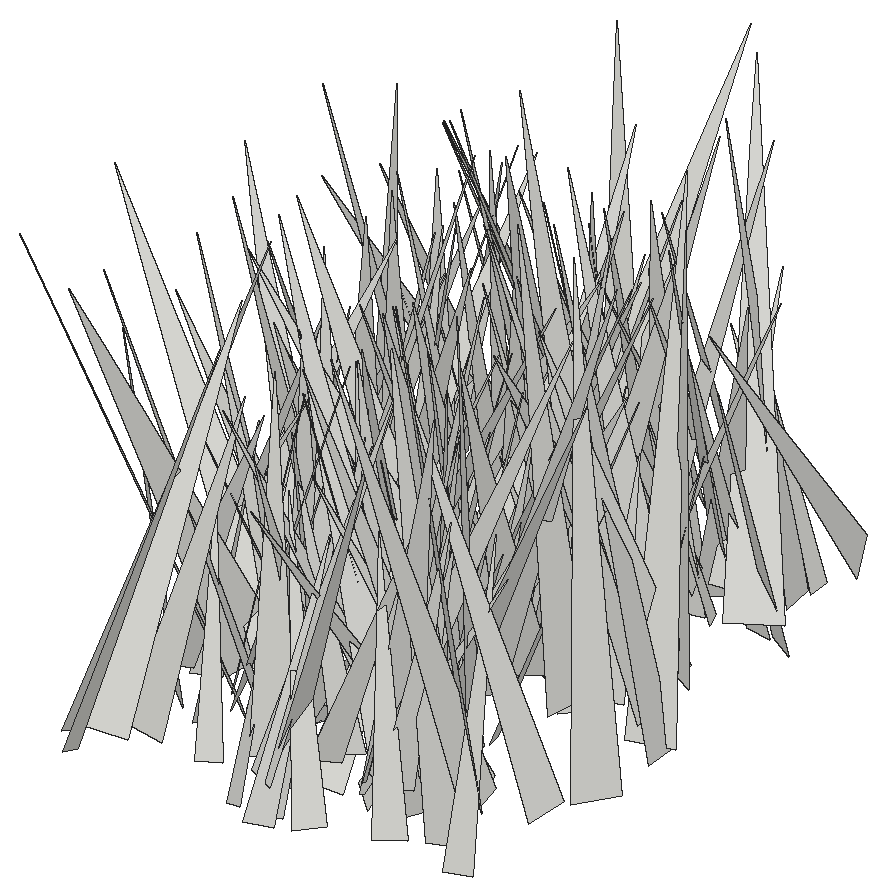
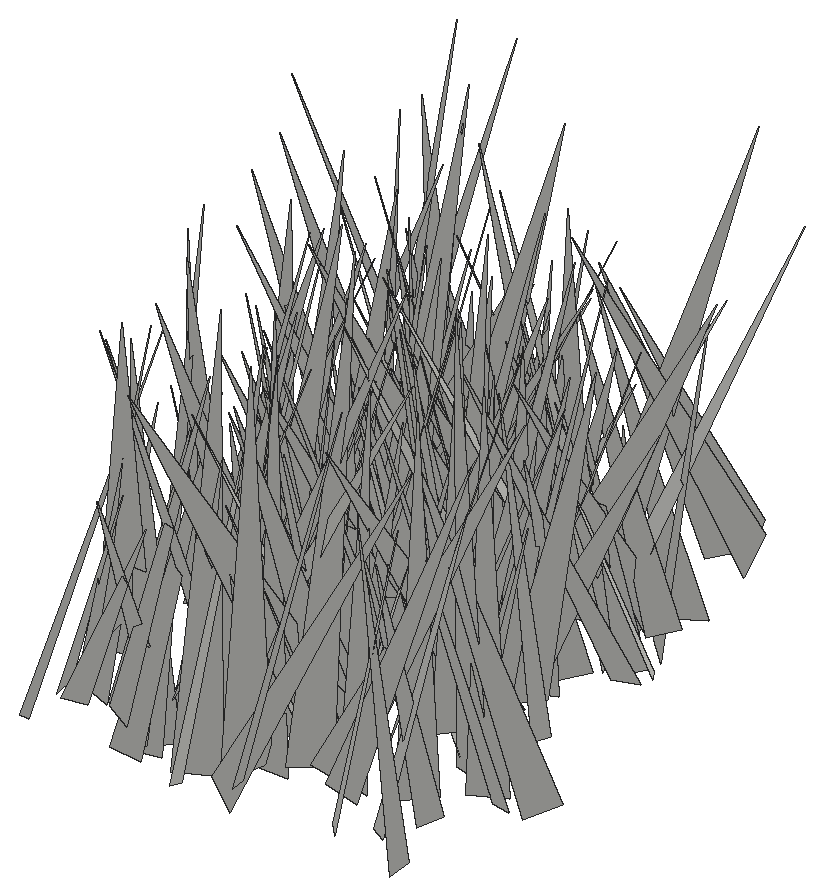
# SketchUp Ruby script. Lengths in inches.
U = 1.inch
M = Sketchup.active_model
def pt(a) = Geom::Point3d.new(a.map { |v| v * U })
def face(e, loops, mat)
  f = e.add_face(loops[0].map { |a| pt(a) })
  loops[1..].each { |l| e.add_face(l.map { |a| pt(a) }).erase! }
  f.material = f.back_material = mat if mat
  f
end
# faces: each face lists its corners as indices into pts; further lists are holes
def faces(e, pts, list, mat = nil) = list.each { |f| face(e, (f[0].is_a?(Array) ? f : [f]).map { |l| l.map { |i| pts[i] } }, mat) }
# xy, xz, yz: faces in a plane at the given z, y or x. An outline is a flat list of corners, or four numbers for a rectangle; further outlines are holes
def ring(l) = l.size == 4 ? [[l[0], l[1]], [l[2], l[1]], [l[2], l[3]], [l[0], l[3]]] : l.each_slice(2).to_a
def flat(e, list, mat, &to3) = list.each { |f| face(e, (f[0].is_a?(Array) ? f : [f]).map { |l| ring(l).map { |u, v| to3.(u, v) } }, mat) }
def xy(e, z, list, mat = nil) = flat(e, list, mat) { |x, y| [x, y, z] }
def xz(e, y, list, mat = nil) = flat(e, list, mat) { |x, z| [x, y, z] }
def yz(e, x, list, mat = nil) = flat(e, list, mat) { |y, z| [x, y, z] }
def lines(e, pts, list) = list.each { |a, b| e.add_line(pt(pts[a]), pt(pts[b])) }
# prism: a flat outline (further loops are holes) pulled along v
def prism(e, loops, v, mat = nil)
  f = face(e, loops, mat); d = Geom::Vector3d.new(v.map { |x| x * U })
  f.pushpull(f.normal.samedirection?(d) ? d.length : -d.length)
end
def box(e, o, s, mat = nil) = prism(e, [[o, [o[0] + s[0], o[1], o[2]], [o[0] + s[0], o[1] + s[1], o[2]], [o[0], o[1] + s[1], o[2]]]], [0, 0, s[2]], mat)
def at(x, y, z, deg = 0) = Geom::Transformation.translation(pt([x, y, z])) * Geom::Transformation.rotation(ORIGIN, Z_AXIS, deg.degrees)
def axes(o, x, y, z) = Geom::Transformation.new([*x, 0, *y, 0, *z, 0, *pt(o).to_a, 1])
def part(name) = M.definitions.add(name)
# library, detail: a bought-in or finely detailed component or shape, given as its bounding box
def library(name, o, s) = part(name).tap { |d| box(d.entities, o, s) }
def detail(e, o, s) = box(e.add_group.entities, o, s)
def put(e, d, t, mat = nil) = e.add_instance(d, t).tap { |i| i.material = mat if mat }
def group(e, t, mat = nil) = e.add_group.tap { |g| g.transformation = t; g.material = mat if mat }.entities
root = M.entities
c1 = part("fur_instance\#9")
p = [[0.8125,0,1.79],[0.67,-0.02,1.48],[0,-0.11,0],[0,0.11,0]]
faces(c1.entities,p,[[0,1,2,3]])
put(root,c1,axes([75.7,109.57,-28.22],[5.32416,0.8497,1.29821],[1.01973,-5.41351,-0.63884],[-1.1694,-0.85204,5.35356]))
put(root,c1,axes([79.16,99.36,-28.22],[-6.20404,3.776,0.73856],[3.82283,6.20814,0.37243],[0.43544,-0.70326,7.25325]))
put(root,c1,axes([79.8125,94.96,-28.22],[-5.60021,-5.8066,0.30959],[-5.79691,5.54128,-0.92996],[-0.45638,0.8674,8.01337]))
put(root,c1,axes([77.96,94.43,-28.22],[-3.7574,-4.18768,1.74578],[-4.4509,3.84178,-0.36412],[0.87968,1.55129,5.61445]))
put(root,c1,axes([79.72,98.95,-28.22],[-2.55985,4.83206,1.74885],[4.89019,1.69025,2.4878],[-1.579,-2.59892,4.86955]))
put(root,c1,axes([77.5,110.44,-27.1],[3.26712,2.26093,2.86418],[3.20778,-3.61207,-0.80776],[-1.73938,-2.41465,3.89016]))
put(root,c1,axes([74.52,104.19,-28.22],[4.53332,-3.78068,0.06575],[-3.6354,-4.32956,1.69931],[1.04008,1.34544,5.65304]))
put(root,c1,axes([77.53,108.27,-28.22],[-3.10311,-4.08719,0.56583],[-3.96021,3.14894,1.02739],[1.15846,-0.18348,5.02781]))
put(root,c1,axes([80.89,95.66,-27.1],[-4.85114,5.94494,0.47809],[5.69058,4.42924,2.66526],[-1.78556,-2.03568,7.19529]))
put(root,c1,axes([76.41,104.47,-28.22],[2.07468,-5.92746,1.15005],[-6.03286,-1.98482,0.6533],[0.24901,1.299,6.24598]))
put(root,c1,axes([78.66,108.61,-27.1],[-0.3519,-5.66898,0.64957],[-5.59847,0.21723,-1.13712],[-1.1029,0.70611,5.5649]))
put(root,c1,axes([76.78,106.73,-28.22],[3.97041,-1.42005,1.05601],[-1.57618,-4.01704,0.5243],[-0.80459,0.86179,4.18399]))
put(root,c1,axes([78.29,102.75,-28.22],[-3.79793,-0.43925,1.06155],[-0.29859,3.91782,0.55288],[1.10936,-0.44932,3.78306]))
put(root,c1,axes([79.55,107.99,-27.1],[1.60402,-6.13136,0.73735],[-5.58582,-1.76536,-2.52831],[-2.63361,0.00991,5.81155]))
put(root,c1,axes([76.08,102.31,-27.1],[5.21952,0.68023,0.61562],[0.83808,-4.98198,-1.60081],[-0.37326,-1.674,5.01433]))
put(root,c1,axes([77.47,103.83,-28.22],[-2.07525,-6.86081,3.30693],[-7.48887,2.46229,0.40886],[1.38687,3.02978,7.15613]))
put(root,c1,axes([75.65,104.77,-28.22],[3.63408,5.21962,1.38175],[5.32326,-3.18476,-1.96987],[0.90365,-2.23003,6.04736]))
put(root,c1,axes([75.9,97.2,-27.1],[3.62695,2.69385,0.06353],[2.59465,-3.4627,-1.30122],[0.7271,-1.08099,4.32648]))
put(root,c1,axes([76.29,98.03,-27.1],[1.18506,6.07091,0.5983],[5.8889,-0.9794,-1.72625],[1.5921,-0.89616,5.93973]))
put(root,c1,axes([77.94,105.9,-28.22],[4.61817,-3.87726,2.02523],[-4.05143,-4.90172,-0.14567],[-1.64942,1.18414,6.02822]))
put(root,c1,axes([78.95,97.17,-28.22],[-3.56448,3.67904,0.44666],[3.56023,3.5714,-1.00507],[1.02934,0.38746,5.02301]))
put(root,c1,axes([79.54,99.4,-27.1],[-6.2182,-2.45212,1.53392],[-2.39925,6.40419,0.51167],[1.61537,0.0727,6.66461]))
put(root,c1,axes([80.97,103.28,-28.22],[-7.24522,-3.15461,1.03201],[-3.28219,7.17812,-1.10079],[0.49381,1.42581,7.82516]))
put(root,c1,axes([77.75,95.9,-28.22],[2.99214,-2.75371,1.44433],[-3.06357,-2.95389,0.71483],[-0.53251,1.52102,4.0031]))
put(root,c1,axes([77.91,105.49,-28.22],[1.29664,4.3065,0.97913],[4.41517,-1.23995,-0.39328],[0.1042,-1.05001,4.48024]))
put(root,c1,axes([78.53,101.6,-27.1],[3.73723,-3.51523,0.8829],[-3.22394,-3.80362,-1.49732],[-1.65607,-0.52811,4.90732]))
put(root,c1,axes([78.18,94.31,-27.1],[5.42222,1.22065,1.50489],[0.3801,-5.05507,2.73075],[-1.90005,2.47215,4.84081]))
put(root,c1,axes([81.82,95.41,-28.22],[-6.83624,-2.0461,0.45627],[-2.08301,6.45462,-2.26447],[-0.23611,2.29788,6.76704]))
put(root,c1,axes([78.0625,89.64,-27.1],[7.02675,2.35333,1.41841],[1.60681,-6.67867,3.12071],[-2.22895,2.60433,6.72121]))
put(root,c1,axes([79.55,95.88,-27.1],[6.1806,-4.85252,1.92283],[-3.89661,-6.27237,-3.30423],[-3.47285,-1.59827,7.12944]))
put(root,c1,axes([79.2,93.72,-28.22],[3.33394,1.47543,1.26624],[0.9738,-3.44268,1.44745],[-1.68284,0.93087,3.34618]))
put(root,c1,axes([78.4,103.62,-27.1],[5.51508,-3.1001,1.56666],[-3.03836,-5.73026,-0.64316],[-1.68328,0.18611,6.29389]))
put(root,c1,axes([78.73,88.67,-27.1],[5.48783,2.36239,1.1528],[1.72376,-5.24883,2.55038],[-1.98455,1.97355,5.40302]))
put(root,c1,axes([82.92,92.9375,-28.22],[-6.43148,-3.95381,0.27263],[-3.76371,5.93049,-2.78112],[-1.24153,2.50351,7.01869]))
put(root,c1,axes([78.77,90.05,-27.1],[-3.2571,5.60614,0.8435],[5.30317,3.35677,-1.83235],[2.00417,0.22864,6.21933]))
put(root,c1,axes([77.24,95.01,-27.1],[3.19208,-3.97574,0.46961],[-3.91795,-2.97897,1.41133],[0.82265,1.2392,4.89939]))
put(root,c1,axes([80.36,101.54,-27.1],[-4.41173,-1.92667,0.46008],[-1.77307,4.34177,1.17998],[0.88316,-0.90777,4.66723]))
put(root,c1,axes([79.1,98.64,-28.22],[1.77747,-4.94769,1.74658],[-5.22789,-1.82695,0.145],[-0.44649,1.69476,5.25529]))
put(root,c1,axes([78.99,100.62,-28.22],[-4.67484,5.38464,0.57126],[4.73589,4.43174,-3.01759],[2.62527,1.59378,6.46085]))
put(root,c1,axes([79.85,101.57,-28.22],[-2.86218,-6.85746,0.77217],[-6.83354,2.93291,0.71683],[0.96112,0.43167,7.39614]))
put(root,c1,axes([78.68,96,-28.22],[4.26525,2.34746,1.0733],[2.44325,-4.34035,-0.2164],[-0.83252,-0.71113,4.86375]))
put(root,c1,axes([80.43,97.98,-27.1],[-5.1029,2.41175,1.4356],[2.37658,5.2976,-0.4521],[1.4931,-0.1897,5.62599]))
put(root,c1,axes([78.4,92.29,-28.22],[-0.20342,5.45726,1.92359],[5.57072,0.70526,-1.41173],[1.56492,-1.80117,5.27542]))
put(root,c1,axes([82.7,109.34,-28.22],[-3.56669,-5.90918,0.59479],[-5.71236,3.22345,-2.22975],[-1.62517,1.63841,6.53207]))
put(root,c1,axes([80.82,105.28,-27.1],[-3.26871,-2.2439,0.63682],[-2.29753,3.28654,-0.21245],[0.40248,0.53729,3.95909]))
put(root,c1,axes([79.03,100.38,-27.1],[3.65147,4.43575,1.22236],[4.5601,-3.69672,-0.20725],[-0.61278,-1.07778,5.74161]))
put(root,c1,axes([79.93,106.5,-28.22],[-1.72933,-6.01967,2.37326],[-6.41752,1.90965,0.16749],[0.82719,2.23073,6.26091]))
put(root,c1,axes([80.49,105.65,-27.1],[-1.33118,-5.02308,1.66852],[-5.29255,1.28443,-0.35575],[0.06525,1.70478,5.18429]))
put(root,c1,axes([81.47,95.4375,-28.22],[0.51311,-4.91857,2.52241],[-5.22585,-1.25725,-1.38854],[-1.80151,2.24614,4.74633]))
put(root,c1,axes([80.88,92.12,-28.22],[-0.87591,3.86506,0.33078],[3.84564,0.82067,0.59405],[-0.50909,-0.4507,3.91829]))
put(root,c1,axes([78.37,103.17,-28.22],[3.8277,2.64651,0.3376],[2.6435,-3.68235,-1.10521],[0.36045,-1.09797,4.52038]))
put(root,c1,axes([82.51,100.73,-28.22],[-5.74656,4.30747,2.03787],[4.75581,5.38477,2.02895],[0.29923,-2.86007,6.88916]))
put(root,c1,axes([80.96,95.77,-27.1],[-0.62514,-3.66803,1.11265],[-3.82799,0.53943,-0.37244],[-0.19721,1.15663,3.70223]))
put(root,c1,axes([82.24,95.56,-27.1],[-2.77092,-3.22119,0.17285],[-3.17409,2.68192,-0.90354],[-0.57541,0.71776,4.15182]))
put(root,c1,axes([81.23,106.09,-27.1],[-3.53133,-2.30027,1.49102],[-2.55807,3.63918,-0.44418],[0.98523,1.20406,4.19097]))
put(root,c1,axes([79.96,101.52,-27.1],[5.42096,2.25752,1.64956],[2.38588,-5.61122,-0.16143],[-1.45775,-0.7887,5.87002]))
put(root,c1,axes([80.29,98.05,-28.22],[6.47169,4.71895,0.84374],[4.29058,-6.33416,2.51645],[-2.13805,1.57262,7.60387]))
put(root,c1,axes([81.28,100.07,-27.1],[0.82489,5.68831,1.342],[5.81529,-0.93413,0.38496],[-0.58339,-1.2684,5.73491]))
put(root,c1,axes([81.42,110.125,-27.1],[-5.10979,-2.8974,1.28802],[-2.4355,5.15064,1.92434],[2.03034,-1.11347,5.54994]))
put(root,c1,axes([84.29,99.72,-27.1],[-7.00038,0.48524,0.02911],[0.47648,6.76613,1.79834],[-0.09628,-1.796,6.78283]))
put(root,c1,axes([83.08,100.31,-27.1],[-4.76571,-0.2474,0.30777],[-0.30187,4.68534,-0.90794],[0.25457,0.92426,4.68496]))
put(root,c1,axes([79.46,101.18,-28.22],[6.355,-3.28716,0.66061],[-3.33311,-6.3472,0.48096],[-0.36352,0.73183,7.13864]))
put(root,c1,axes([80.43,107.92,-27.1],[7.22069,-3.00234,1.05262],[-2.62839,-7.10035,-2.22196],[-1.79266,-1.6827,7.49769]))
put(root,c1,axes([84.94,106.07,-27.1],[-4.9499,-5.12629,0.49866],[-4.98162,4.58947,-2.26921],[-1.30806,1.92014,6.75508]))
put(root,c1,axes([81.72,94.61,-27.1],[5.15692,6.28398,0.1894],[5.87834,-4.90651,2.73667],[-2.22922,1.59869,7.6546]))
put(root,c1,axes([82.65,97.14,-28.22],[-4.87312,1.26006,1.29377],[1.19613,5.04128,-0.40455],[1.35309,0.08157,5.01711]))
put(root,c1,axes([84.2,103.88,-27.1],[-6.46812,-3.13785,1.21731],[-3.3431,6.29489,-1.53709],[0.38946,1.92167,7.02282]))
put(root,c1,axes([82.96,107.8,-28.22],[-7.16118,3.19135,1.99245],[3.1192,7.43157,-0.69239],[2.1036,-0.15533,7.80947]))
put(root,c1,axes([82,104.25,-28.22],[-2.04424,6.85145,0.72305],[6.79433,2.1298,-0.97223],[1.1412,-0.40704,7.08351]))
put(root,c1,axes([80.88,94.08,-27.1],[4.18181,1.0835,0.53294],[1.13424,-4.18373,-0.39425],[-0.41412,-0.51766,4.30187]))
put(root,c1,axes([80.7,100.6,-27.1],[0.16634,-6.6201,0.01552],[-6.42128,-0.15757,1.61124],[1.61035,0.05552,6.42319]))
put(root,c1,axes([84.9375,100.1,-28.22],[-7.26619,-2.16018,0.91047],[-2.32448,7.02333,-1.88745],[0.30351,2.07347,7.34176]))
put(root,c1,axes([78.87,104.51,-27.1],[4.45492,4.83666,0.95124],[4.56601,-3.56591,-3.25273],[1.85733,-2.83468,5.71483]))
put(root,c1,axes([82.91,90.64,-28.22],[1.74005,3.73475,0.21366],[3.48509,-1.70407,1.40429],[-1.35946,0.41179,3.87351]))
put(root,c1,axes([81.61,96.42,-28.22],[-1.23587,-5.65616,0.92472],[-5.5483,1.41785,1.25724],[1.43652,0.61007,5.65145]))
put(root,c1,axes([80.42,93.99,-27.1],[6.04949,2.12455,0.78775],[2.22415,-5.99674,-0.90711],[-0.43293,-1.1207,6.34722]))
put(root,c1,axes([85.12,106.41,-28.22],[-4.28269,-7.03673,0.88853],[-7.06243,4.13524,-1.29164],[-0.65353,1.42504,8.13564]))
put(root,c1,axes([82.52,95.08,-27.1],[0.52075,4.40411,1.27547],[4.58416,-0.47433,-0.2338],[0.09203,-1.29345,4.42863]))
put(root,c1,axes([82.72,104.97,-27.1],[1.79845,4.31058,0.12569],[4.2592,-1.79684,0.67963],[-0.67534,0.14702,4.621]))
put(root,c1,axes([81.63,100.59,-28.22],[4.69401,2.26049,0.88712],[2.32694,-4.7392,-0.23643],[-0.69438,-0.60059,5.20458]))
put(root,c1,axes([81.97,106.84,-27.1],[0.88242,4.55252,0.64978],[4.54635,-0.76413,-0.82042],[0.6916,-0.78549,4.5641]))
put(root,c1,axes([83.24,91.96,-27.1],[3.99343,-3.31881,2.86458],[-3.84361,-4.5142,0.12826],[-2.10878,1.94301,5.19091]))
put(root,c1,axes([80.8,104.46,-28.22],[5.6454,-1.61471,0.55375],[-1.70236,-5.46688,1.41409],[-0.12614,1.5134,5.69896]))
put(root,c1,axes([82.5,102.02,-27.1],[3.11347,-5.57932,0.56956],[-5.54553,-3.1599,-0.63956],[-0.83685,0.18197,6.35716]))
put(root,c1,axes([80.24,106.49,-28.22],[5.01746,5.30698,2.27397],[5.71554,-4.13917,-2.95123],[0.81705,-3.63499,6.68051]))
put(root,c1,axes([82.65,94.89,-27.1],[5.01646,-0.03484,2.02413],[0.79085,-4.94522,-2.0451],[-1.86357,-2.19241,4.58078]))
put(root,c1,axes([83.53,97.5,-27.1],[-6.08575,-1.31512,1.93305],[-0.80976,6.24223,1.69745],[2.19329,-1.34444,5.99037]))
put(root,c1,axes([82.76,104.67,-27.1],[-6.00676,5.62271,0.83771],[4.81686,5.68135,-3.59416],[3.01902,2.12255,7.40122]))
put(root,c1,axes([82.41,105.54,-28.22],[3.10796,2.24348,0.34109],[2.21254,-3.12436,0.38987],[-0.50422,0.11876,3.81322]))
put(root,c1,axes([83.4375,97.15,-28.22],[3.82096,-4.05561,2.24215],[-4.19487,-4.26194,-0.56033],[-1.96935,1.20949,5.5438]))
put(root,c1,axes([82.32,107.34,-28.22],[-1.45623,-6.82166,1.9418],[-6.84757,1.86878,1.42991],[1.84835,1.54881,6.82723]))
put(root,c1,axes([85.27,95.02,-27.1],[-5.50457,-1.9976,0.13924],[-1.94432,5.42927,1.02602],[0.47897,-0.91798,5.76524]))
put(root,c1,axes([82.47,103.81,-27.1],[4.37125,-4.19897,0.80164],[-4.19734,-4.43318,-0.33332],[-0.81017,0.31203,6.05212]))
put(root,c1,axes([82.51,100.48,-27.1],[-2.22642,5.28944,0.76409],[4.89566,2.35054,-2.00661],[2.14349,0.12554,5.37668]))
put(root,c1,axes([84.88,93.32,-27.1],[0.57769,-3.84784,2.16026],[-4.16363,-1.197,-1.01866],[-1.46176,1.88882,3.75525]))
put(root,c1,axes([84.28,100.22,-27.1],[-5.52668,-3.91053,1.22579],[-3.5737,5.60606,1.77193],[2.00587,-0.78663,6.53427]))
put(root,c1,axes([86.04,94.11,-27.1],[-6.89397,4.20656,1.53795],[4.42912,6.82252,1.19307],[0.66584,-1.82904,7.9874]))
put(root,c1,axes([83.04,99.23,-27.1],[4.10361,0.18993,0.89205],[0.09258,-4.17709,0.46346],[-0.90734,0.43277,4.08178]))
put(root,c1,axes([84.08,90.7,-28.22],[-4.0426,1.99311,1.15136],[1.52694,4.06338,-1.67276],[1.72237,1.07573,4.18533]))
put(root,c1,axes([83.54,102.59,-28.22],[4.6203,4.92142,0.32663],[4.69042,-4.52255,1.79463],[-1.52544,1.00021,6.50745]))
put(root,c1,axes([84.06,107.27,-28.22],[4.90048,2.76624,3.25214],[3.64641,-5.28694,-0.99757],[-2.22086,-2.5767,5.5382]))
put(root,c1,axes([85.4,90.9,-28.22],[-4.1604,2.35856,0.20079],[2.33408,4.15517,-0.44576],[0.39395,0.28953,4.76162]))
put(root,c1,axes([84.16,90.2,-28.22],[-3.28423,2.60896,0.74342],[2.31234,3.30268,-1.37511],[1.4186,0.65664,3.96257]))
put(root,c1,axes([84.45,95.87,-27.1],[-3.67064,-4.64361,1.03864],[-4.58105,3.8034,0.81465],[1.28682,0.29416,5.86285]))
put(root,c1,axes([82.9,111.23,-27.1],[-3.72735,-5.65721,0.3773],[-4.71825,3.34531,3.54775],[3.14396,-1.68653,5.77153]))
put(root,c1,axes([84.38,107.97,-28.22],[-2.15861,-6.19615,1.53511],[-6.31129,2.3146,0.46773],[0.95736,1.28794,6.5447]))
put(root,c1,axes([86.4,101.65,-27.1],[-5.31837,-1.43549,0.4315],[-1.49067,5.23198,-0.96754],[0.15722,1.04767,5.42306]))
put(root,c1,axes([83.34,105.8,-27.1],[3.34183,1.38887,0.77255],[1.56239,-3.2005,-1.00466],[-0.29109,-1.23347,3.4767]))
put(root,c1,axes([82.01,95.97,-28.22],[7.35163,-0.33714,0.71191],[-0.54127,-7.01692,2.26646],[-0.57229,2.30568,7.00167]))
put(root,c1,axes([84.17,92.95,-28.22],[-2.9389,4.8588,0.20427],[4.55933,2.83593,-1.85926],[1.6918,0.79774,5.36547]))
put(root,c1,axes([83.84,90.6875,-27.1],[2.91229,5.1803,0.24137],[5.15397,-2.92189,0.52374],[-0.57474,0.04729,5.91968]))
put(root,c1,axes([86.36,102.61,-27.1],[-0.9931,7.68396,2.84346],[8.04191,0.36629,1.81887],[-1.56723,-2.98953,7.53135]))
put(root,c1,axes([86.34,95.8,-28.22],[0.43766,-5.35462,0.13989],[-4.92597,-0.45748,-2.09965],[-2.10387,-0.04276,4.94519]))
put(root,c1,axes([84.03,108.82,-28.22],[3.11086,-6.46121,1.0779],[-6.53922,-3.13316,0.09147],[-0.38422,1.01124,7.17051]))
put(root,c1,axes([84.11,101.77,-27.1],[-0.58036,-3.55618,1.37675],[-3.59236,0.97706,1.00942],[1.27936,1.13031,3.45894]))
put(root,c1,axes([83.19,101.02,-28.22],[6.28882,0.29269,0.74734],[0.08478,-6.11246,1.68051],[-0.79813,1.65699,6.06719]))
put(root,c1,axes([86.3,106.9,-27.1],[-5.06216,-2.56794,0.53616],[-2.44101,5.03776,1.08155],[0.96086,-0.73072,5.57226]))
put(root,c1,axes([86.0625,106.88,-28.22],[-0.90978,-4.59674,2.27002],[-5.08569,0.51819,-0.98893],[-0.64715,2.39002,4.58036]))
put(root,c1,axes([84.5,101.92,-28.22],[2.70818,5.99392,1.73773],[6.22026,-2.74585,-0.22279],[-0.5051,-1.67756,6.57356]))
put(root,c1,axes([86.28,104.52,-28.22],[-3.5972,0.42819,0.55364],[0.48536,3.61469,0.35791],[0.50428,-0.42464,3.60487]))
put(root,c1,axes([82.58,102.59,-28.22],[2.62599,-5.06265,0.78885],[-4.77605,-2.09765,2.43674],[1.85526,1.76578,5.15641]))
put(root,c1,axes([85.58,101.91,-27.1],[3.95748,1.9361,2.48086],[2.44941,-4.39763,-0.47534],[-1.97573,-1.57388,4.37997]))
put(root,c1,axes([84.89,95.41,-27.1],[0.96438,4.41888,0.40988],[4.43511,-0.94495,-0.24768],[0.15571,-0.45288,4.5161]))
put(root,c1,axes([83.59,91.67,-28.22],[6.64605,0.23955,0.93352],[0.28653,-6.70181,-0.32012],[-0.92019,-0.35664,6.64266]))
put(root,c1,axes([86.23,105.08,-27.1],[-2.52047,3.62206,0.22803],[3.61381,2.53037,-0.24846],[0.33426,-0.04477,4.40572]))
put(root,c1,axes([84.68,103.71,-27.1],[6.67924,-1.26552,2.75336],[-2.18749,-6.62541,2.26131],[-2.097,2.88046,6.41095]))
put(root,c1,axes([88.34,93.79,-27.1],[-1.48445,-5.73193,2.26963],[-5.6541,0.33538,-2.85107],[-2.45713,2.69116,5.18942]))
put(root,c1,axes([86.75,107.03,-28.22],[-3.24657,-1.58505,0.39086],[-1.61743,3.24104,-0.29141],[0.22149,0.43432,3.60107]))
put(root,c1,axes([84.99,98.57,-27.1],[5.51708,-5.76072,0.82028],[-5.55442,-5.55067,-1.6234],[-1.73412,-0.54876,7.80952]))
put(root,c1,axes([87.88,103.19,-27.1],[-6.93734,1.12272,0.61983],[1.08478,6.95591,-0.45824],[0.68406,0.3553,7.01265]))
put(root,c1,axes([86.95,103.69,-27.1],[-5.18557,-4.32883,1.54546],[-4.49087,5.26797,-0.31293],[0.97941,1.23577,6.74766]))
put(root,c1,axes([86.71,101.73,-28.22],[0.84597,-3.78981,1.14812],[-3.67965,-1.18614,-1.20406],[-1.46323,0.79177,3.69169]))
put(root,c1,axes([85.6,102.3125,-28.22],[-2.42915,2.39744,1.43013],[2.49267,2.71628,-0.31959],[1.25681,-0.75355,3.39799]))
put(root,c1,axes([85.32,100.76,-27.1],[3.56693,3.32971,1.1246],[3.34181,-3.70943,0.38354],[-1.08812,-0.47732,4.86445]))
put(root,c1,axes([87.78,95.7,-28.22],[-5.4104,-1.19331,0.05848],[-1.15989,5.3113,1.06983],[0.28647,-1.03242,5.43616]))
put(root,c1,axes([86.2,92.34,-27.1],[3.78632,3.0497,0.88341],[2.42458,-3.66486,2.25998],[-2.05,1.29824,4.30457]))
put(root,c1,axes([84.27,97.18,-28.22],[2.24479,3.42751,0.35228],[3.3467,-2.06895,-1.19586],[0.81948,-0.93948,3.91878]))
put(root,c1,axes([86.8,109.09,-27.1],[-2.84226,-5.05917,1.08036],[-5.16298,2.85167,-0.22901],[0.32566,1.05526,5.79838]))
put(root,c1,axes([84.99,105.81,-28.22],[2.96798,6.81466,1.03357],[6.887,-2.97737,-0.1458],[-0.27767,-1.00619,7.4315]))
put(root,c1,axes([87.11,96.17,-27.1],[-3.42512,-4.29344,1.99666],[-4.721,3.28594,-1.03273],[0.36395,2.21827,5.39431]))
put(root,c1,axes([84.59,92.59,-27.1],[3.70527,-2.55389,0.75103],[-2.66189,-3.54115,1.0909],[0.02774,1.32414,4.36593]))
put(root,c1,axes([85.41,98.65,-27.1],[1.48907,3.83094,1.46531],[4.09712,-1.31638,-0.722],[0.19182,-1.62223,4.04625]))
put(root,c1,axes([86.43,109.2,-28.22],[-0.49515,-5.81147,0.35136],[-5.82208,0.49376,-0.03799],[-0.0081,0.35331,5.8324]))
put(root,c1,axes([85.875,96.02,-28.22],[5.47086,1.91538,2.35531],[2.21322,-5.83902,-0.39241],[-2.07794,-1.17628,5.78316]))
put(root,c1,axes([86.98,100.5625,-28.22],[-3.68366,1.92684,0.76086],[1.83141,3.75443,-0.64122],[0.96827,0.22919,4.10742]))
put(root,c1,axes([86.31,104.47,-27.1],[4.64507,-4.79979,0.2726],[-4.36308,-4.36804,-2.56373],[-2.01887,-1.6035,6.16782]))
put(root,c1,axes([85.93,99.9,-27.1],[3.11864,-5.68803,0.55795],[-5.6529,-3.16353,-0.65398],[-0.84244,0.17118,6.45383]))
put(root,c1,axes([86.47,92.58,-27.1],[3.93079,5.90323,1.06815],[5.73682,-4.07234,1.39466],[-1.7544,-0.09002,6.95371]))
put(root,c1,axes([87.07,107.08,-27.1],[0.03105,4.61747,0.04613],[4.59439,-0.03553,0.46309],[-0.46341,-0.04278,4.59429]))
put(root,c1,axes([84.81,100.49,-28.22],[3.88446,1.51086,0.00017],[1.46105,-3.75628,-1.06181],[0.38475,-0.98965,4.03042]))
put(root,c1,axes([84.82,97.47,-27.1],[6.67299,1.88656,0.54903],[1.75109,-6.59185,1.3677],[-0.89119,1.17381,6.79833]))
put(root,c1,axes([90.02,100.14,-27.1],[-7.1325,-1.97369,0.04131],[-1.9512,7.0246,-1.27181],[-0.29997,1.23662,7.29044]))
put(root,c1,axes([87.55,91.77,-28.22],[-2.17723,3.86998,1.04919],[4.00343,2.16477,0.32287],[0.22393,-1.07466,4.42864]))
put(root,c1,axes([88.39,109.1875,-27.1],[-2.47066,2.78913,0.64805],[2.82871,2.24449,1.12431],[-0.44456,-1.21919,3.55237]))
put(root,c1,axes([87.15,93.23,-28.22],[5.18015,0.30458,2.40247],[-0.20645,-5.59667,1.15468],[-2.41288,1.13276,5.059]))
put(root,c1,axes([86.27,97.95,-28.22],[4.68389,2.5085,0.46697],[2.25732,-4.52881,1.68637],[-1.1896,1.28326,5.03861]))
put(root,c1,axes([89.02,106,-27.1],[-3.36629,7.35026,0.38103],[7.33966,3.3212,0.77612],[-0.54849,-0.66835,8.0471]))
put(root,c1,axes([87.94,99.26,-27.1],[-7.15931,0.95304,2.49675],[1.12982,7.54938,0.35801],[2.42189,-0.70454,7.21359]))
put(root,c1,axes([88.65,93.52,-28.22],[-4.01127,-3.66818,1.32519],[-3.89401,3.87381,-1.06408],[0.2199,1.68524,5.33044]))
put(root,c1,axes([88.2,107.24,-28.22],[-1.41742,-4.71426,1.18858],[-4.85717,1.31918,-0.56008],[-0.21176,1.29675,4.89077]))
put(root,c1,axes([89.12,107.81,-27.1],[-6.73527,-1.87686,1.53677],[-2.12146,6.75676,-1.04577],[1.17629,1.43931,6.91323]))
put(root,c1,axes([85.79,108.75,-28.22],[-3.7888,-7.35051,1.42507],[-6.56657,4.02946,3.32556],[3.59735,-0.38635,7.57137]))
put(root,c1,axes([85.68,98.13,-27.1],[6.84778,-1.68967,1.39359],[-1.92956,-6.81846,1.21431],[-1.03628,1.53061,6.94784]))
put(root,c1,axes([85.96,93.73,-28.22],[4.71855,-5.46855,1.25045],[-5.59838,-4.69426,0.59612],[-0.35606,1.33873,7.19821]))
put(root,c1,axes([85.43,93.23,-28.22],[2.80072,3.68056,0.20092],[3.50306,-2.57922,-1.58339],[1.14693,-1.10998,4.34551]))
put(root,c1,axes([89.04,92.56,-28.22],[-0.80473,7.1427,2.6366],[7.51279,0.31449,1.44102],[-1.23607,-2.73867,7.04196]))
put(root,c1,axes([86.97,93.29,-27.1],[3.29573,-2.04708,1.27302],[-2.29025,-3.33183,0.57152],[-0.75223,1.17531,3.83742]))
put(root,c1,axes([85.1875,105.55,-28.22],[5.31801,3.62577,0.57345],[3.65614,-5.14142,-1.39812],[0.32822,-1.47507,6.28273]))
put(root,c1,axes([86.03,108.15,-28.22],[4.15858,-4.6502,0.45845],[-4.67236,-4.14601,0.32855],[-0.05962,0.56087,6.22978]))
put(root,c1,axes([87.39,101.625,-28.22],[-1.6026,3.32948,1.45838],[3.48573,1.8596,-0.41502],[1.03054,-1.11225,3.67172]))
put(root,c1,axes([87.14,92.55,-27.1],[3.46953,-2.67132,1.40146],[-2.94376,-3.4648,0.68347],[-0.65905,1.41311,4.3251]))
put(root,c1,axes([89.18,108.68,-27.1],[-3.86057,-0.50737,0.50019],[-0.53854,3.88252,-0.21837],[0.46646,0.28336,3.88764]))
put(root,c1,axes([90.45,100.17,-28.22],[-7.60093,-1.69118,1.08047],[-1.85126,7.54274,-1.21718],[0.77483,1.43129,7.69108]))
put(root,c1,axes([87.5,93.52,-27.1],[-3.93965,-2.75758,3.63418],[-3.8658,4.56754,-0.72493],[2.42222,2.80458,4.7539]))
put(root,c1,axes([88.79,93.99,-27.1],[-6.27895,-2.5321,2.5957],[-2.9165,6.61067,-0.60625],[2.15482,1.56906,6.74309]))
put(root,c1,axes([89.13,102.15,-27.1],[5.01755,-2.86523,2.69296],[-2.1597,-5.65647,-1.99435],[-3.28592,-0.6574,5.42291]))
put(root,c1,axes([89.56,93.25,-27.1],[-7.48109,-1.28394,1.71532],[-0.94889,7.57103,1.5286],[1.92105,-1.26035,7.43496]))
put(root,c1,axes([85.54,93.72,-27.1],[3.97232,6.71602,1.21655],[6.692,-3.55551,-2.22255],[1.34242,-2.14887,7.47961]))
put(root,c1,axes([89.78,100.47,-28.22],[-0.32528,8.12923,0.88129],[8.06717,0.17507,1.36272],[-1.33486,-0.92294,8.0208]))
put(root,c1,axes([89.16,93.56,-27.1],[-5.20637,-5.83633,2.28098],[-6.06397,5.44004,0.07832],[1.57922,1.64775,7.82067]))
put(root,c1,axes([90.57,97.1,-28.22],[-7.32985,2.37013,1.25415],[2.21242,7.40801,-1.06942],[1.51512,0.64882,7.62892]))
put(root,c1,axes([89.36,102.3,-27.1],[3.04497,5.63186,2.55497],[5.93211,-3.46487,0.56775],[-1.7481,-1.94792,6.3771]))
put(root,c1,axes([86.6,94.97,-27.1],[6.73911,-0.51973,0.37006],[-0.5475,-6.72675,0.52311],[-0.32757,0.55072,6.73884]))
put(root,c1,axes([90.18,91.46,-28.22],[-4.48023,1.71415,0.10108],[1.53614,4.12726,-1.90446],[0.76734,1.74596,4.4027]))
put(root,c1,axes([91.1875,94.14,-27.1],[-6.42244,0.41118,0.57395],[0.45958,6.42194,0.54196],[0.53597,-0.57954,6.41273]))
put(root,c1,axes([88.04,102.64,-27.1],[3.15545,2.01724,0.79775],[2.15051,-3.09372,-0.68323],[-0.2846,-1.01105,3.6823]))
put(root,c1,axes([89.17,107.02,-28.22],[-1.94034,-4.30134,0.80925],[-4.30819,2.03312,0.47669],[0.77193,0.53502,4.69459]))
put(root,c1,axes([88.97,110.85,-27.1],[-5.2943,-3.28141,1.0592],[-2.29433,4.80125,3.40634],[2.57403,-2.46971,5.21479]))
